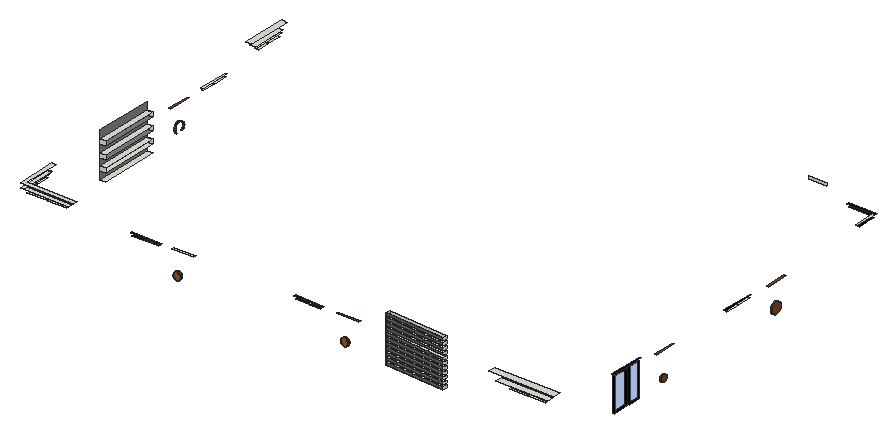
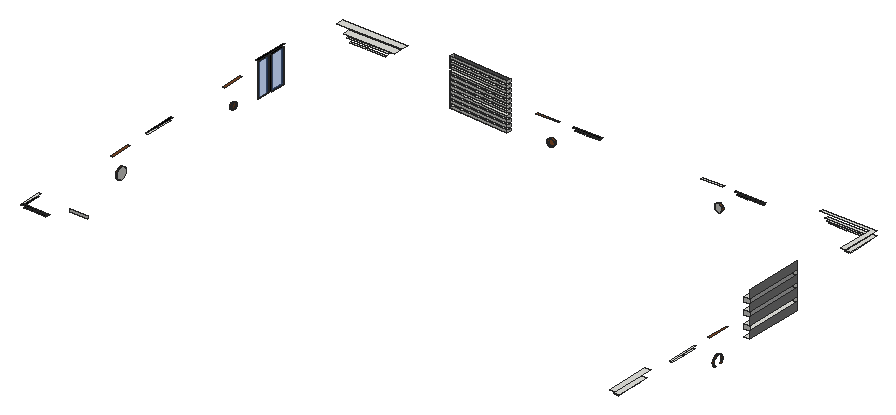
# SketchUp Ruby script. Lengths in inches.
U = 1.inch
M = Sketchup.active_model
def pt(a) = Geom::Point3d.new(a.map { |v| v * U })
def face(e, loops, mat)
  f = e.add_face(loops[0].map { |a| pt(a) })
  loops[1..].each { |l| e.add_face(l.map { |a| pt(a) }).erase! }
  f.material = f.back_material = mat if mat
  f
end
# faces: each face lists its corners as indices into pts; further lists are holes
def faces(e, pts, list, mat = nil) = list.each { |f| face(e, (f[0].is_a?(Array) ? f : [f]).map { |l| l.map { |i| pts[i] } }, mat) }
# xy, xz, yz: faces in a plane at the given z, y or x. An outline is a flat list of corners, or four numbers for a rectangle; further outlines are holes
def ring(l) = l.size == 4 ? [[l[0], l[1]], [l[2], l[1]], [l[2], l[3]], [l[0], l[3]]] : l.each_slice(2).to_a
def flat(e, list, mat, &to3) = list.each { |f| face(e, (f[0].is_a?(Array) ? f : [f]).map { |l| ring(l).map { |u, v| to3.(u, v) } }, mat) }
def xy(e, z, list, mat = nil) = flat(e, list, mat) { |x, y| [x, y, z] }
def xz(e, y, list, mat = nil) = flat(e, list, mat) { |x, z| [x, y, z] }
def yz(e, x, list, mat = nil) = flat(e, list, mat) { |y, z| [x, y, z] }
def lines(e, pts, list) = list.each { |a, b| e.add_line(pt(pts[a]), pt(pts[b])) }
# prism: a flat outline (further loops are holes) pulled along v
def prism(e, loops, v, mat = nil)
  f = face(e, loops, mat); d = Geom::Vector3d.new(v.map { |x| x * U })
  f.pushpull(f.normal.samedirection?(d) ? d.length : -d.length)
end
def box(e, o, s, mat = nil) = prism(e, [[o, [o[0] + s[0], o[1], o[2]], [o[0] + s[0], o[1] + s[1], o[2]], [o[0], o[1] + s[1], o[2]]]], [0, 0, s[2]], mat)
def at(x, y, z, deg = 0) = Geom::Transformation.translation(pt([x, y, z])) * Geom::Transformation.rotation(ORIGIN, Z_AXIS, deg.degrees)
def axes(o, x, y, z) = Geom::Transformation.new([*x, 0, *y, 0, *z, 0, *pt(o).to_a, 1])
def part(name) = M.definitions.add(name)
# library, detail: a bought-in or finely detailed component or shape, given as its bounding box
def library(name, o, s) = part(name).tap { |d| box(d.entities, o, s) }
def detail(e, o, s) = box(e.add_group.entities, o, s)
def put(e, d, t, mat = nil) = e.add_instance(d, t).tap { |i| i.material = mat if mat }
def group(e, t, mat = nil) = e.add_group.tap { |g| g.transformation = t; g.material = mat if mat }.entities
root = M.entities
M.materials.add("[0133_Gray]").color = [128, 128, 128]
M.materials.add("[0134_DimGray]").color = [105, 105, 105]
M.materials.add("[0137_Black]").color = [0, 0, 0]
M.materials.add("[Translucent Glass Blue]").color = [100, 149, 237]
M.materials["[Translucent Glass Blue]"].alpha = 0.5
M.materials.add("[Wood Cherry Original]").color = [152, 86, 42]
M.materials.add("[Wood Veneer 01]").color = [120, 70, 37]
xy(root,534.54,[[972.47,237.17,975.47,262.14],[972.47,266.68,975.47,287.11]],"[0137_Black]")
xy(root,535.48,[[766.05,146.53,667.69,152.53,668.06,158.52,766.41,152.52]])
xy(root,539.68,[[766.05,146.53,766.41,152.52,668.06,158.52,667.69,152.53]])
xy(root,539.88,[[83.8125,295.24,92.8125,392.06]])
xy(root,542.73,[[766.05,146.53,667.69,152.53,668.06,158.52,766.41,152.52]])
xy(root,546.93,[[766.05,146.53,766.41,152.52,668.06,158.52,667.69,152.53]])
xy(root,549.98,[[766.05,146.53,667.69,152.53,668.06,158.52,766.41,152.52]])
xy(root,552.37,[[83.8125,295.24,92.8125,392.06]])
xy(root,554.18,[[766.05,146.53,766.41,152.52,668.06,158.52,667.69,152.53]])
xy(root,557.23,[[766.05,146.53,667.69,152.53,668.06,158.52,766.41,152.52]])
xy(root,559.81,[[83.8125,295.24,92.8125,392.06]])
xy(root,561.43,[[766.05,146.53,766.41,152.52,668.06,158.52,667.69,152.53]])
xy(root,564.48,[[766.05,146.53,667.69,152.53,668.06,158.52,766.41,152.52]])
xy(root,568.68,[[766.05,146.53,766.41,152.52,668.06,158.52,667.69,152.53]])
xy(root,571.73,[[766.05,146.53,667.69,152.53,668.06,158.52,766.41,152.52]])
xy(root,572.31,[[83.8125,295.24,92.8125,392.06]],"[0133_Gray]")
xy(root,573.58,[[872.2,149.58,901.73,152.58],[904.37,149.58,931.26,152.58]])
xy(root,575.93,[[766.05,146.53,766.41,152.52,668.06,158.52,667.69,152.53]])
xy(root,576.7,[[248.3125,155.58,269.91,158.58],[272.57,155.58,291.5,158.58]],"[0137_Black]")
xy(root,577.48,[[80.8125,508.73,83.8125,527.36],[80.8125,530.57,83.8125,552.41]])
xy(root,577.89,[[517.1,155.58,537.51,158.58],[540.34,155.58,557.92,158.58]],"[0137_Black]")
xy(root,578.98,[[766.05,146.53,667.69,152.53,668.06,158.52,766.41,152.52]])
xy(root,579.13,[[866.65,149.58,936.8125,152.58]])
xy(root,579.7,[[245.3125,155.58,294.5,158.58]],"[0137_Black]")
xy(root,579.75,[[83.8125,295.24,92.8125,392.06]])
xy(root,580.06,[[80.8125,440.49,83.8125,476.49]],"[Wood Veneer 01]")
xy(root,580.47,[[313.74,155.58,349.74,158.58]])
xy(root,580.47,[[584.77,155.58,620.77,158.58]],"[Wood Cherry Original]")
xy(root,580.48,[[80.8125,505.73,83.8125,555.41]])
xy(root,580.89,[[514.1,155.58,560.92,158.58]],"[0137_Black]")
xy(root,582.56,[[972.47,552.41,975.47,588.41]],"[Wood Veneer 01]")
xy(root,582.79,[[972.47,467.5,975.47,490.72],[972.47,493.16,975.47,513.9375]])
xy(root,582.97,[[74.8125,628.16,77.8125,647],[74.8125,649.88,77.8125,671.6]])
xy(root,583.1,[[857.16,140.58,941.79,152.58]])
xy(root,583.18,[[766.05,146.53,766.41,152.52,668.06,158.52,667.69,152.53]])
xy(root,583.19,[[972.47,322.375,975.47,358.375]],"[Wood Veneer 01]")
xy(root,583.79,[[80.8125,149.58,112.875,152.58],[114.7,149.58,144.9375,152.58],[74.8125,155.58,77.8125,172.52],[74.8125,175.24,77.8125,194.89]])
xy(root,585.79,[[972.47,464.5,975.47,516.9375]],"[0137_Black]")
xy(root,586.23,[[766.05,146.53,667.69,152.53,668.06,158.52,766.41,152.52]])
xy(root,586.31,[[74.8125,624.83,77.8125,674.93]])
xy(root,586.79,[[74.8125,149.58,147.9375,152.58],[74.8125,152.58,77.8125,197.89]])
xy(root,588.98,[[71.8125,146.58,71.8125,203.77,77.8125,203.77,77.8125,152.58,151.54,152.58,151.54,146.58]])
xy(root,589.47,[[972.47,738.61,975.47,753.05],[972.47,755.68,975.47,767.48],[933.09,770.48,948.82,773.48],[951.28,770.48,969.47,773.48]],"[0137_Black]")
xy(root,589.49,[[68.8125,621.65,77.8125,678.11]])
xy(root,589.54,[[972.47,237.17,975.47,262.14],[972.47,266.68,975.47,287.11]],"[0137_Black]")
xy(root,590.43,[[766.05,146.53,766.41,152.52,668.06,158.52,667.69,152.53]])
xy(root,592.25,[[83.8125,295.24,92.8125,392.06]],"[0133_Gray]")
xy(root,592.47,[[972.47,735.61,975.47,770.48]])
xy(root,592.47,[[930.09,770.48,972.47,773.48],[972.47,770.48,975.47,773.48]],"[0137_Black]")
xy(root,592.54,[[972.47,234.17,975.47,290.11]],"[0137_Black]")
xy(root,593.48,[[766.05,146.53,667.69,152.53,668.06,158.52,766.41,152.52]])
xy(root,593.76,[[846.5,140.58,952.45,152.58]])
xy(root,596.48,[[71.8125,146.58,159.375,146.58,159.375,152.58,77.8125,152.58,77.8125,211.02,71.8125,211.02]])
xy(root,597.29,[[68.8125,613.85,77.8125,685.91]])
xy(root,597.68,[[766.05,146.53,766.41,152.52,668.06,158.52,667.69,152.53]])
xy(root,599.69,[[83.8125,295.24,92.8125,392.06]])
xy(root,600.73,[[766.05,146.53,667.69,152.53,668.06,158.52,766.41,152.52]])
xy(root,604.93,[[766.05,146.53,766.41,152.52,668.06,158.52,667.69,152.53]])
xy(root,607.98,[[766.05,146.53,667.69,152.53,668.06,158.52,766.41,152.52]])
xz(root,152.58,[[599.13,537.91,600.73,538.12,602.22,538.73,603.5,539.72,604.49,541,605.11,542.49,605.32,544.09,605.11,545.69,604.49,547.1875,603.5,548.47,602.22,549.45,600.73,550.07,599.13,550.28,597.53,550.07,596.04,549.45,594.75,548.47,593.77,547.1875,593.15,545.69,592.94,544.09,593.15,542.49,593.77,541,594.75,539.72,596.04,538.73,597.53,538.12],[323.72,538.36,325.35,538.45,326.9,538.96,328.27,539.85,329.36,541.07,330.09,542.52,330.43,544.12,330.33,545.75,329.82,547.3,328.93,548.66,327.72,549.75,326.26,550.49,324.66,550.82,323.03,550.73,321.48,550.22,320.12,549.33,319.03,548.11,318.29,546.65,317.96,545.06,318.05,543.43,318.5625,541.88,319.45,540.51,320.67,539.43,322.125,538.6875]],"[Wood Cherry Original]")
xz(root,155.58,[[323.72,538.36,322.125,538.6875,320.67,539.43,319.45,540.51,318.5625,541.88,318.05,543.43,317.96,545.06,318.29,546.65,319.03,548.11,320.12,549.33,321.48,550.22,323.03,550.73,324.66,550.82,326.26,550.49,327.72,549.75,328.93,548.66,329.82,547.3,330.33,545.75,330.43,544.12,330.09,542.52,329.36,541.07,328.27,539.85,326.9,538.96,325.35,538.45]])
xz(root,203.77,[[71.8125,588.98,77.8125,589.29]])
xz(root,237.17,[[972.47,534.54,975.47,589.54]],"[0137_Black]")
xz(root,262.14,[[972.47,534.54,975.47,589.54]],"[0137_Black]")
xz(root,266.68,[[972.47,534.54,975.47,589.54]],"[0137_Black]")
xz(root,287.11,[[972.47,534.54,975.47,589.54]],"[0137_Black]")
xz(root,295.24,[[83.8125,552.37,92.8125,559.81],[83.8125,572.31,92.8125,579.75],[83.8125,592.25,92.8125,599.69]])
xz(root,392.06,[[83.8125,552.37,92.8125,559.81],[83.8125,572.31,92.8125,579.75],[83.8125,592.25,92.8125,599.69]])
xz(root,770.48,[[866.95,607.37,896.3125,612.18]])
yz(root,83.8125,[[295.24,539.88,392.06,552.37],[295.24,559.81,392.06,572.31],[295.24,579.75,392.06,592.25],[295.24,599.69,392.06,612.18]],"[0133_Gray]")
yz(root,972.47,[[237.17,534.54,262.14,589.54],[266.68,534.54,287.11,589.54]],"[Translucent Glass Blue]")
yz(root,975.47,[[565.29,537.46,562.96,537.77,560.79,538.67,558.93,540.1,557.5,541.96,556.6,544.13,556.29,546.46,556.6,548.79,557.5,550.96,558.93,552.83,560.79,554.26,562.96,555.16,565.29,555.46,567.62,555.16,569.79,554.26,571.65,552.83,573.08,550.96,573.98,548.79,574.29,546.46,573.98,544.13,573.08,541.96,571.65,540.1,569.79,538.67,567.62,537.77]])
yz(root,978.47,[[565.29,537.46,567.62,537.77,569.79,538.67,571.65,540.1,573.08,541.96,573.98,544.13,574.29,546.46,573.98,548.79,573.08,550.96,571.65,552.83,569.79,554.26,567.62,555.16,565.29,555.46,562.96,555.16,560.79,554.26,558.93,552.83,557.5,550.96,556.6,548.79,556.29,546.46,556.6,544.13,557.5,541.96,558.93,540.1,560.79,538.67,562.96,537.77],[334.56,539.19,335.9,539.37,337.15,539.89,338.23,540.71,339.05,541.79,339.57,543.04,339.75,544.38,339.57,545.72,339.05,546.97,338.23,548.05,337.15,548.875,335.9,549.39,334.56,549.57,333.22,549.39,331.97,548.875,330.89,548.05,330.07,546.97,329.55,545.72,329.37,544.38,329.55,543.04,330.07,541.79,330.89,540.71,331.97,539.89,333.22,539.37]],"[Wood Veneer 01]")
p = [[80.8125,456.54,535.01],[80.8125,455.11,536.88],[77.8125,455.11,536.88],[77.8125,456.54,535.01],[80.8125,470.7,536.88],[80.8125,469.27,535.01],
  [77.8125,469.27,535.01],[77.8125,470.7,536.88],[766.05,146.53,539.68],[667.69,152.53,539.68],[667.69,152.53,535.48],[766.05,146.53,535.48],
  [766.41,152.52,535.48],[766.41,152.52,539.68],[668.06,158.52,539.68],[668.06,158.52,535.48],[80.8125,454.21,539.05],[77.8125,454.21,539.05],
  [80.8125,471.6,539.05],[77.8125,471.6,539.05],[975.47,562.96,537.77],[975.47,565.29,537.46],[978.47,565.29,537.46],[978.47,562.96,537.77],
  [975.47,567.62,537.77],[978.47,567.62,537.77],[975.47,560.79,538.67],[978.47,560.79,538.67],[975.47,569.79,538.67],[978.47,569.79,538.67],
  [597.53,155.58,538.12],[599.13,155.58,537.91],[599.13,152.58,537.91],[597.53,152.58,538.12],[600.73,155.58,538.12],[600.73,152.58,538.12],
  [596.04,155.58,538.73],[596.04,152.58,538.73],[602.22,155.58,538.73],[602.22,152.58,538.73],[322.125,155.58,538.6875],[323.72,155.58,538.36],
  [323.72,152.58,538.36],[322.125,152.58,538.6875],[325.35,155.58,538.45],[325.35,152.58,538.45],[326.9,155.58,538.96],[326.9,152.58,538.96],
  [320.67,155.58,539.43],[320.67,152.58,539.43],[594.75,155.58,539.72],[594.75,152.58,539.72],[603.5,155.58,539.72],[603.5,152.58,539.72],
  [975.47,558.93,540.1],[978.47,558.93,540.1],[975.47,571.65,540.1],[978.47,571.65,540.1],[328.27,155.58,539.85],[328.27,152.58,539.85],
  [80.8125,453.9,541.38],[77.8125,453.9,541.38],[80.8125,471.9,541.38],[77.8125,471.9,541.38],[975.47,333.22,539.37],[975.47,334.56,539.19],
  [978.47,334.56,539.19],[978.47,333.22,539.37],[975.47,335.9,539.37],[978.47,335.9,539.37],[319.45,155.58,540.51],[319.45,152.58,540.51],
  [975.47,331.97,539.89],[978.47,331.97,539.89],[975.47,337.15,539.89],[978.47,337.15,539.89],[593.77,155.58,541],[593.77,152.58,541],
  [604.49,155.58,541],[604.49,152.58,541],[329.36,155.58,541.07],[329.36,152.58,541.07],[975.47,330.89,540.71],[978.47,330.89,540.71],
  [975.47,338.23,540.71],[978.47,338.23,540.71],[975.47,557.5,541.96],[978.47,557.5,541.96],[975.47,573.08,541.96],[978.47,573.08,541.96],
  [318.5625,155.58,541.88],[318.5625,152.58,541.88],[975.47,330.07,541.79],[978.47,330.07,541.79],[975.47,339.05,541.79],[978.47,339.05,541.79],
  [593.15,155.58,542.49],[593.15,152.58,542.49],[605.11,155.58,542.49],[605.11,152.58,542.49],[330.09,155.58,542.52],[330.09,152.58,542.52],
  [80.8125,454.21,543.71],[77.8125,454.21,543.71],[80.8125,471.6,543.71],[77.8125,471.6,543.71],[975.47,329.55,543.04],[978.47,329.55,543.04],
  [975.47,339.57,543.04],[978.47,339.57,543.04],[318.05,155.58,543.43],[318.05,152.58,543.43],[975.47,556.6,544.13],[978.47,556.6,544.13],
  [975.47,573.98,544.13],[978.47,573.98,544.13],[330.43,155.58,544.12],[330.43,152.58,544.12],[592.94,155.58,544.09],[592.94,152.58,544.09],
  [605.32,155.58,544.09],[605.32,152.58,544.09],[766.05,146.53,546.93],[667.69,152.53,546.93],[667.69,152.53,542.73],[766.05,146.53,542.73],
  [766.41,152.52,542.73],[766.41,152.52,546.93],[668.06,158.52,546.93],[668.06,158.52,542.73],[975.47,329.37,544.38],[978.47,329.37,544.38],
  [975.47,339.75,544.38],[978.47,339.75,544.38],[317.96,155.58,545.06],[317.96,152.58,545.06],[80.8125,455.11,545.88],[77.8125,455.11,545.88],
  [80.8125,470.7,545.88],[77.8125,470.7,545.88],[330.33,155.58,545.75],[330.33,152.58,545.75],[593.15,155.58,545.69],[593.15,152.58,545.69],
  [605.11,155.58,545.69],[605.11,152.58,545.69],[975.47,556.29,546.46],[978.47,556.29,546.46],[975.47,574.29,546.46],[978.47,574.29,546.46],
  [975.47,329.55,545.72],[978.47,329.55,545.72],[975.47,339.57,545.72],[978.47,339.57,545.72],[318.29,155.58,546.65],[318.29,152.58,546.65],
  [329.82,155.58,547.3],[329.82,152.58,547.3],[593.77,155.58,547.1875],[593.77,152.58,547.1875],[604.49,155.58,547.1875],[604.49,152.58,547.1875],
  [975.47,330.07,546.97],[978.47,330.07,546.97],[975.47,339.05,546.97],[978.47,339.05,546.97],[80.8125,456.54,547.74],[77.8125,456.54,547.74],
  [80.8125,469.27,547.74],[77.8125,469.27,547.74],[975.47,556.6,548.79],[978.47,556.6,548.79],[975.47,573.98,548.79],[978.47,573.98,548.79],
  [319.03,155.58,548.11],[319.03,152.58,548.11],[975.47,330.89,548.05],[978.47,330.89,548.05],[975.47,338.23,548.05],[978.47,338.23,548.05],
  [594.75,155.58,548.47],[594.75,152.58,548.47],[603.5,155.58,548.47],[603.5,152.58,548.47],[328.93,155.58,548.66],[328.93,152.58,548.66],
  [80.8125,458.4,549.17],[77.8125,458.4,549.17],[80.8125,467.4,549.17],[77.8125,467.4,549.17],[975.47,331.97,548.875],[978.47,331.97,548.875],
  [975.47,337.15,548.875],[978.47,337.15,548.875],[320.12,155.58,549.33],[320.12,152.58,549.33],[596.04,155.58,549.45],[596.04,152.58,549.45],
  [602.22,155.58,549.45],[602.22,152.58,549.45],[327.72,155.58,549.75],[327.72,152.58,549.75],[975.47,557.5,550.96],[978.47,557.5,550.96],
  [975.47,573.08,550.96],[978.47,573.08,550.96],[975.47,333.22,549.39],[978.47,333.22,549.39],[975.47,335.9,549.39],[978.47,335.9,549.39],
  [80.8125,460.57,550.07],[77.8125,460.57,550.07],[80.8125,465.23,550.07],[77.8125,465.23,550.07],[321.48,155.58,550.22],[321.48,152.58,550.22],
  [975.47,334.56,549.57],[978.47,334.56,549.57],[597.53,155.58,550.07],[597.53,152.58,550.07],[600.73,155.58,550.07],[600.73,152.58,550.07],
  [326.26,155.58,550.49],[326.26,152.58,550.49],[766.05,146.53,554.18],[667.69,152.53,554.18],[667.69,152.53,549.98],[766.05,146.53,549.98],
  [766.41,152.52,549.98],[766.41,152.52,554.18],[668.06,158.52,554.18],[668.06,158.52,549.98],[599.13,155.58,550.28],[599.13,152.58,550.28],
  [80.8125,462.9,550.38],[77.8125,462.9,550.38],[323.03,155.58,550.73],[323.03,152.58,550.73],[324.66,155.58,550.82],[324.66,152.58,550.82],
  [975.47,558.93,552.83],[978.47,558.93,552.83],[975.47,571.65,552.83],[978.47,571.65,552.83],[975.47,560.79,554.26],[978.47,560.79,554.26],
  [975.47,569.79,554.26],[978.47,569.79,554.26],[975.47,562.96,555.16],[978.47,562.96,555.16],[975.47,567.62,555.16],[978.47,567.62,555.16],
  [975.47,565.29,555.46],[978.47,565.29,555.46],[766.05,146.53,561.43],[667.69,152.53,561.43],[667.69,152.53,557.23],[766.05,146.53,557.23],
  [766.41,152.52,557.23],[766.41,152.52,561.43],[668.06,158.52,561.43],[668.06,158.52,557.23],[766.05,146.53,568.68],[667.69,152.53,568.68],
  [667.69,152.53,564.48],[766.05,146.53,564.48],[766.41,152.52,564.48],[766.41,152.52,568.68],[668.06,158.52,568.68],[668.06,158.52,564.48],
  [766.05,146.53,575.93],[667.69,152.53,575.93],[667.69,152.53,571.73],[766.05,146.53,571.73],[766.41,152.52,571.73],[766.41,152.52,575.93],
  [668.06,158.52,575.93],[668.06,158.52,571.73],[766.05,146.53,583.18],[667.69,152.53,583.18],[667.69,152.53,578.98],[766.05,146.53,578.98],
  [766.41,152.52,578.98],[766.41,152.52,583.18],[668.06,158.52,583.18],[668.06,158.52,578.98],[766.05,146.53,590.43],[667.69,152.53,590.43],
  [667.69,152.53,586.23],[766.05,146.53,586.23],[766.41,152.52,586.23],[766.41,152.52,590.43],[668.06,158.52,590.43],[668.06,158.52,586.23],
  [766.05,146.53,597.68],[667.69,152.53,597.68],[667.69,152.53,593.48],[766.05,146.53,593.48],[766.41,152.52,593.48],[766.41,152.52,597.68],
  [668.06,158.52,597.68],[668.06,158.52,593.48],[766.05,146.53,604.93],[667.69,152.53,604.93],[667.69,152.53,600.73],[766.05,146.53,600.73],
  [766.41,152.52,600.73],[766.41,152.52,604.93],[668.06,158.52,604.93],[668.06,158.52,600.73],[668.06,152.51,612.18],[667.69,152.53,612.18],
  [667.69,152.53,607.98],[766.05,146.53,607.98],[766.05,146.53,612.18],[766.41,152.52,607.98],[766.41,152.52,612.18],[668.06,158.52,612.18],
  [668.06,158.52,607.98],[667.69,152.58,612.18],[77.8125,203.77,589.29],[77.8125,146.58,589.29]]
faces(root,p,[[0,1,2,3],[4,5,6,7],[1,16,17,2],[18,4,7,19],[20,21,22,23],[21,24,25,22],[26,20,23,27],[24,28,29,25],
  [54,26,27,55],[28,56,57,29],[16,60,61,17],[62,18,19,63],[64,65,66,67],[65,68,69,66],[72,64,67,73],[68,74,75,69],
  [82,72,73,83],[74,84,85,75],[86,54,55,87],[56,88,89,57],[92,82,83,93],[84,94,95,85],[60,102,103,61],[104,62,63,105],
  [106,92,93,107],[94,108,109,95],[112,86,87,113],[88,114,115,89],[130,106,107,131],[108,132,133,109],[102,136,137,103],[138,104,105,139],
  [146,112,113,147],[114,148,149,115],[150,130,131,151],[132,152,153,133],[162,150,151,163],[152,164,165,153],[136,166,167,137],[168,138,139,169],
  [170,146,147,171],[148,172,173,149],[176,162,163,177],[164,178,179,165],[166,186,187,167],[188,168,169,189],[190,176,177,191],[178,192,193,179],
  [202,170,171,203],[172,204,205,173],[206,190,191,207],[192,208,209,193],[186,210,211,187],[212,188,189,213],[216,206,207,217],[208,216,217,209],
  [210,234,235,211],[234,212,213,235],[240,202,203,241],[204,242,243,205],[244,240,241,245],[242,246,247,243],[248,244,245,249],[246,250,251,247],
  [252,248,249,253],[250,252,253,251]],"[Wood Veneer 01]")
faces(root,p,[[8,9,10,11],[122,123,124,125],[224,225,226,227],[254,255,256,257],[262,263,264,265],[270,271,272,273],[278,279,280,281],[286,287,288,289],
  [294,295,296,297],[302,303,304,305],[310,311,312,313,314]],"[0134_DimGray]")
faces(root,p,[[12,13,8,11],[14,15,10,9],[14,13,12,15],[126,127,122,125],[128,129,124,123],[128,127,126,129],[228,229,224,227],[230,231,226,225],
  [230,229,228,231],[258,259,254,257],[260,261,256,255],[260,259,258,261],[266,267,262,265],[268,269,264,263],[268,267,266,269],[274,275,270,273],
  [276,277,272,271],[276,275,274,277],[282,283,278,281],[284,285,280,279],[284,283,282,285],[290,291,286,289],[292,293,288,287],[292,291,290,293],
  [298,299,294,297],[300,301,296,295],[300,299,298,301],[306,307,302,305],[308,309,304,303],[308,307,306,309],[315,316,314,313],[317,318,312,311,319],
  [317,316,315,318]])
faces(root,p,[[30,31,32,33],[31,34,35,32],[36,30,33,37],[34,38,39,35],[40,41,42,43],[41,44,45,42],[44,46,47,45],[48,40,43,49],
  [50,36,37,51],[38,52,53,39],[46,58,59,47],[70,48,49,71],[76,50,51,77],[52,78,79,53],[58,80,81,59],[90,70,71,91],
  [96,76,77,97],[78,98,99,79],[80,100,101,81],[110,90,91,111],[100,116,117,101],[118,96,97,119],[98,120,121,99],[134,110,111,135],
  [116,140,141,117],[142,118,119,143],[120,144,145,121],[154,134,135,155],[140,156,157,141],[158,142,143,159],[144,160,161,145],[174,154,155,175],
  [180,158,159,181],[160,182,183,161],[156,184,185,157],[194,174,175,195],[196,180,181,197],[182,198,199,183],[184,200,201,185],[214,194,195,215],
  [218,196,197,219],[198,220,221,199],[200,222,223,201],[232,218,219,233],[220,232,233,221],[236,214,215,237],[222,238,239,223],[238,236,237,239]],"[Wood Cherry Original]")
lines(root,p,[[320,321]])
